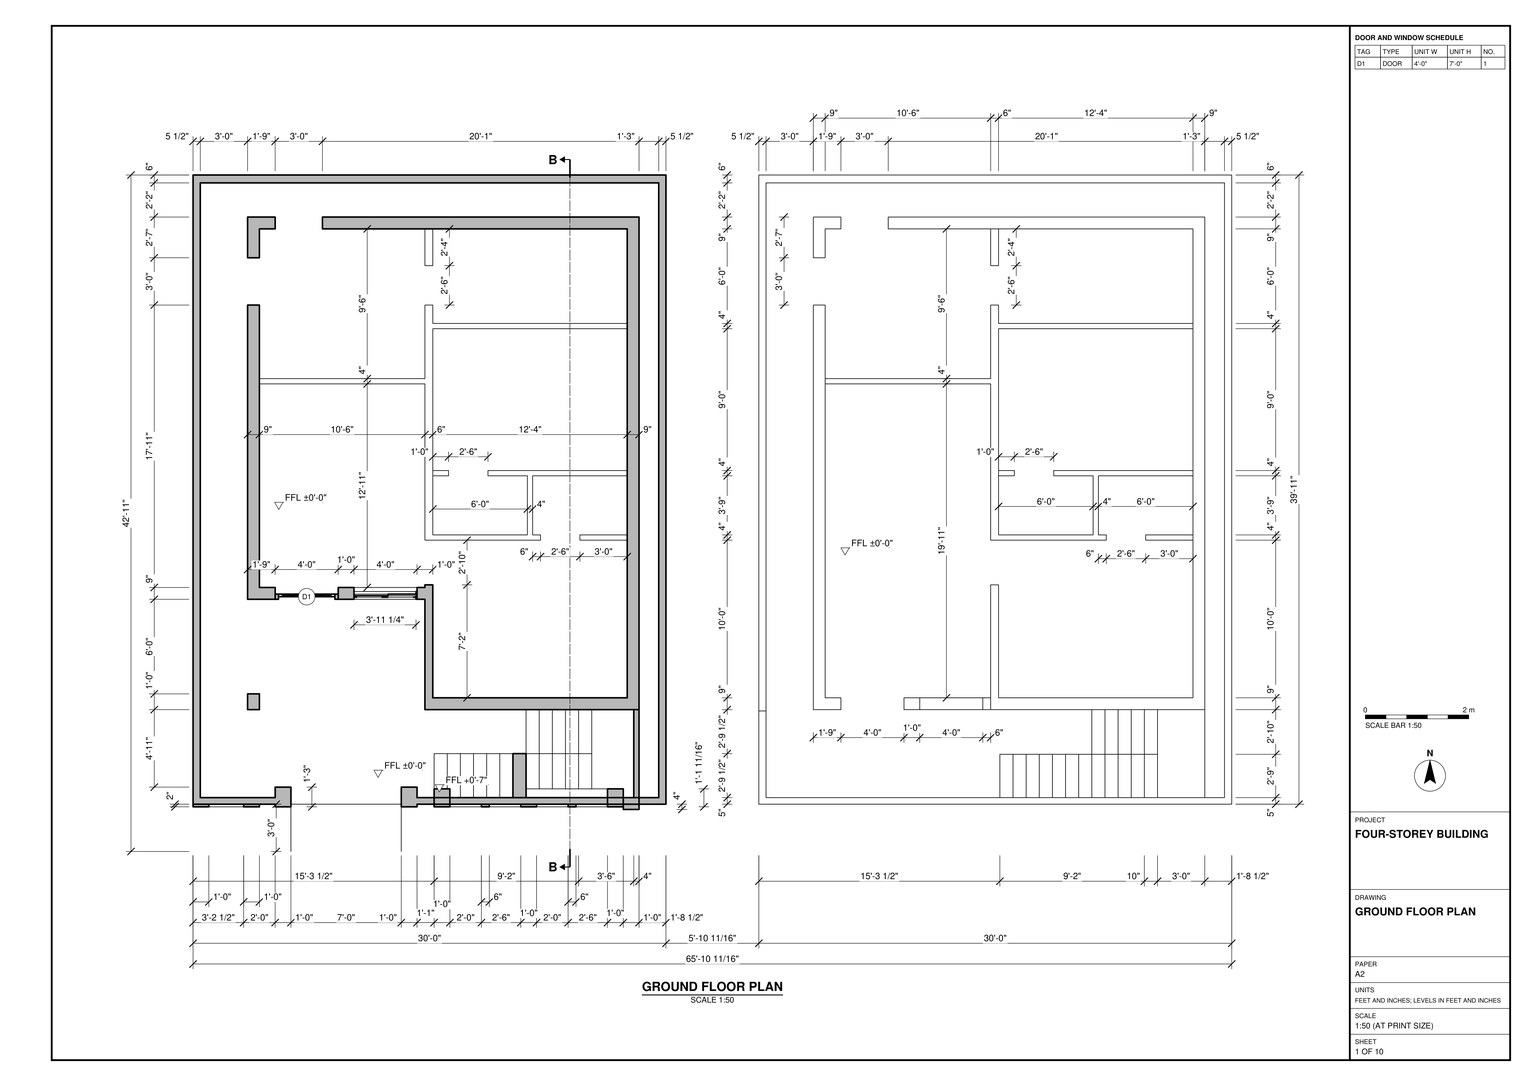
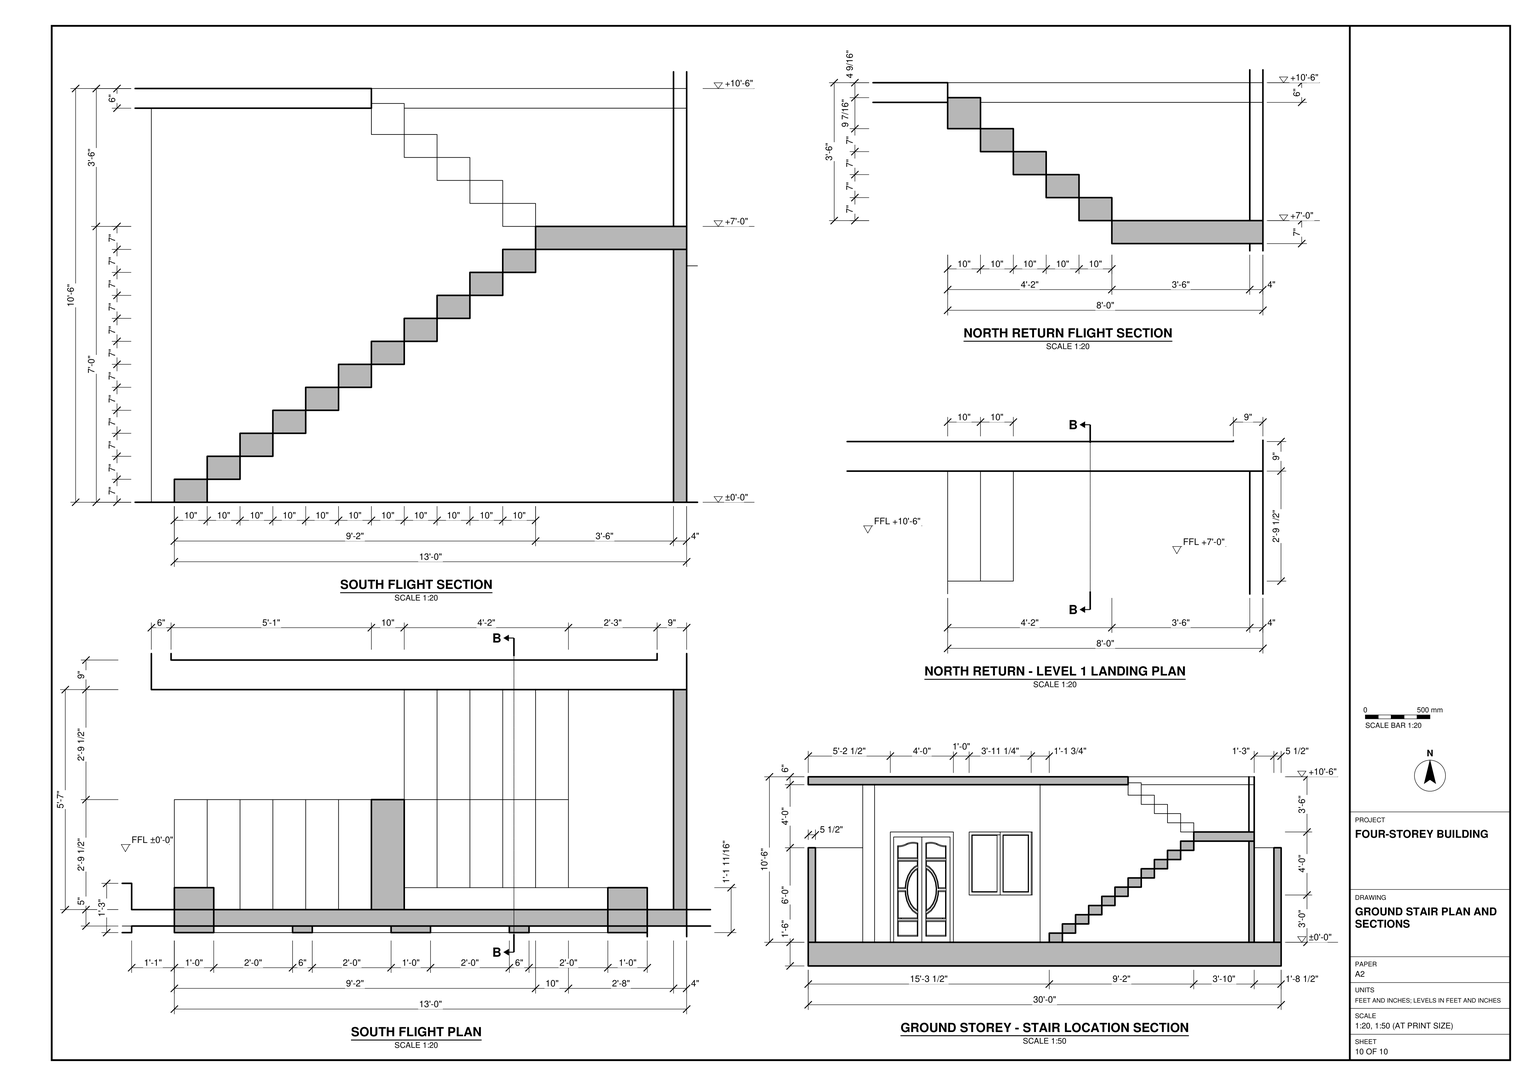
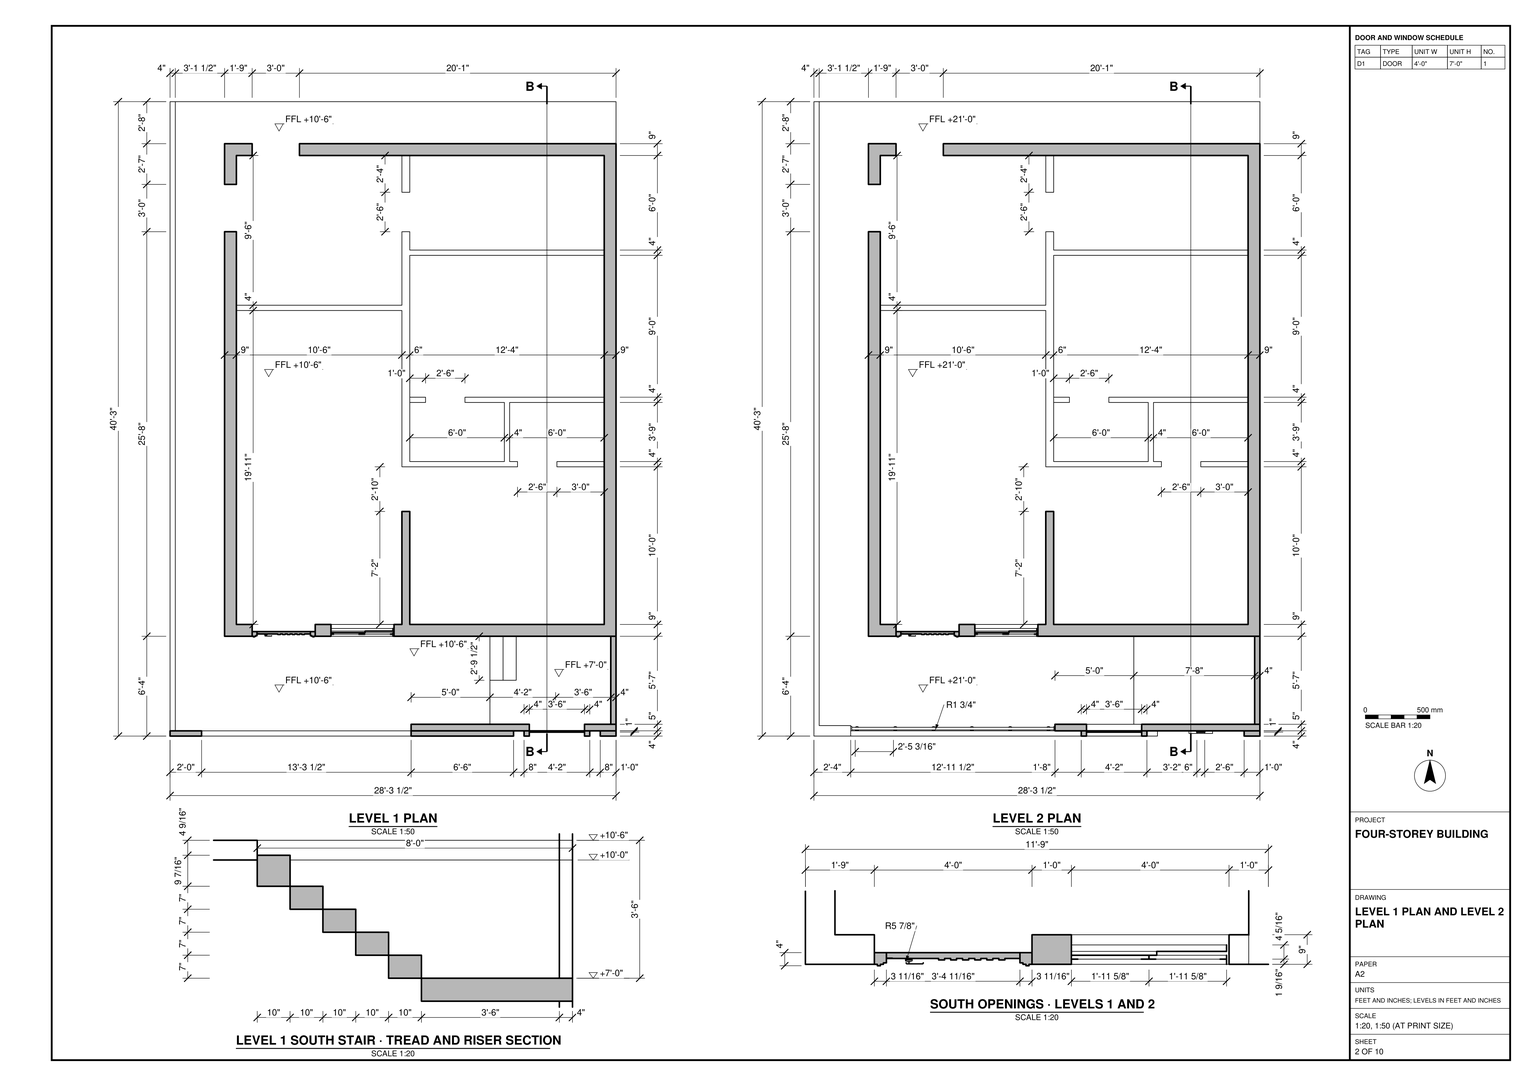
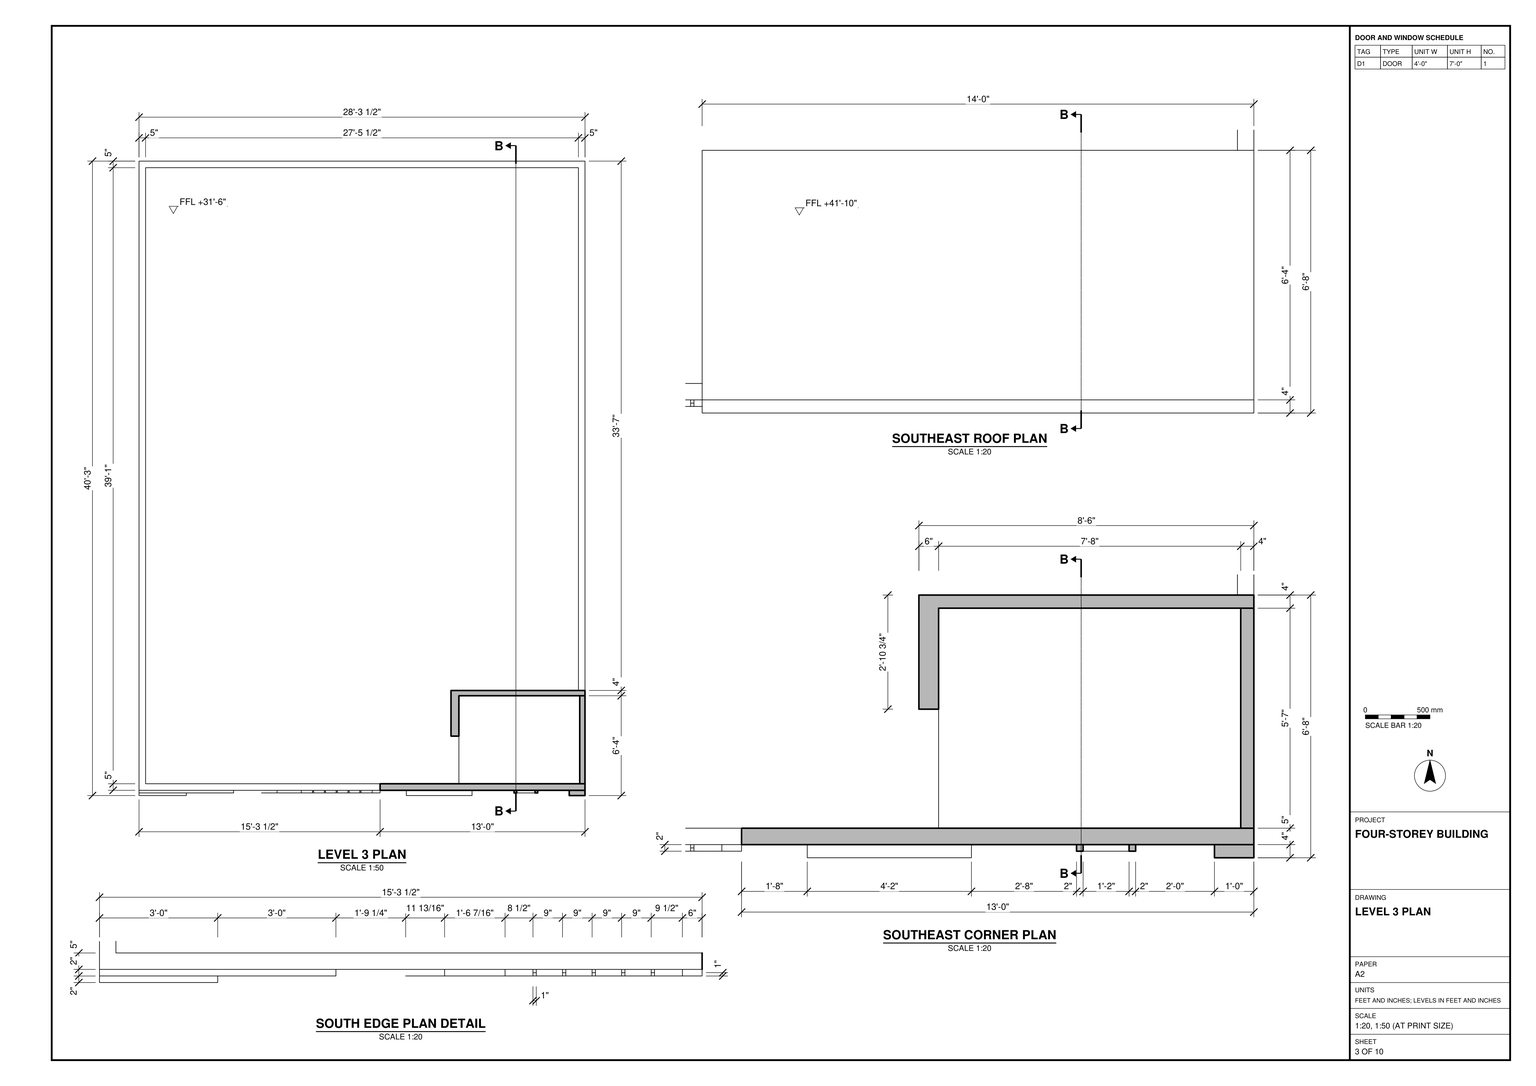
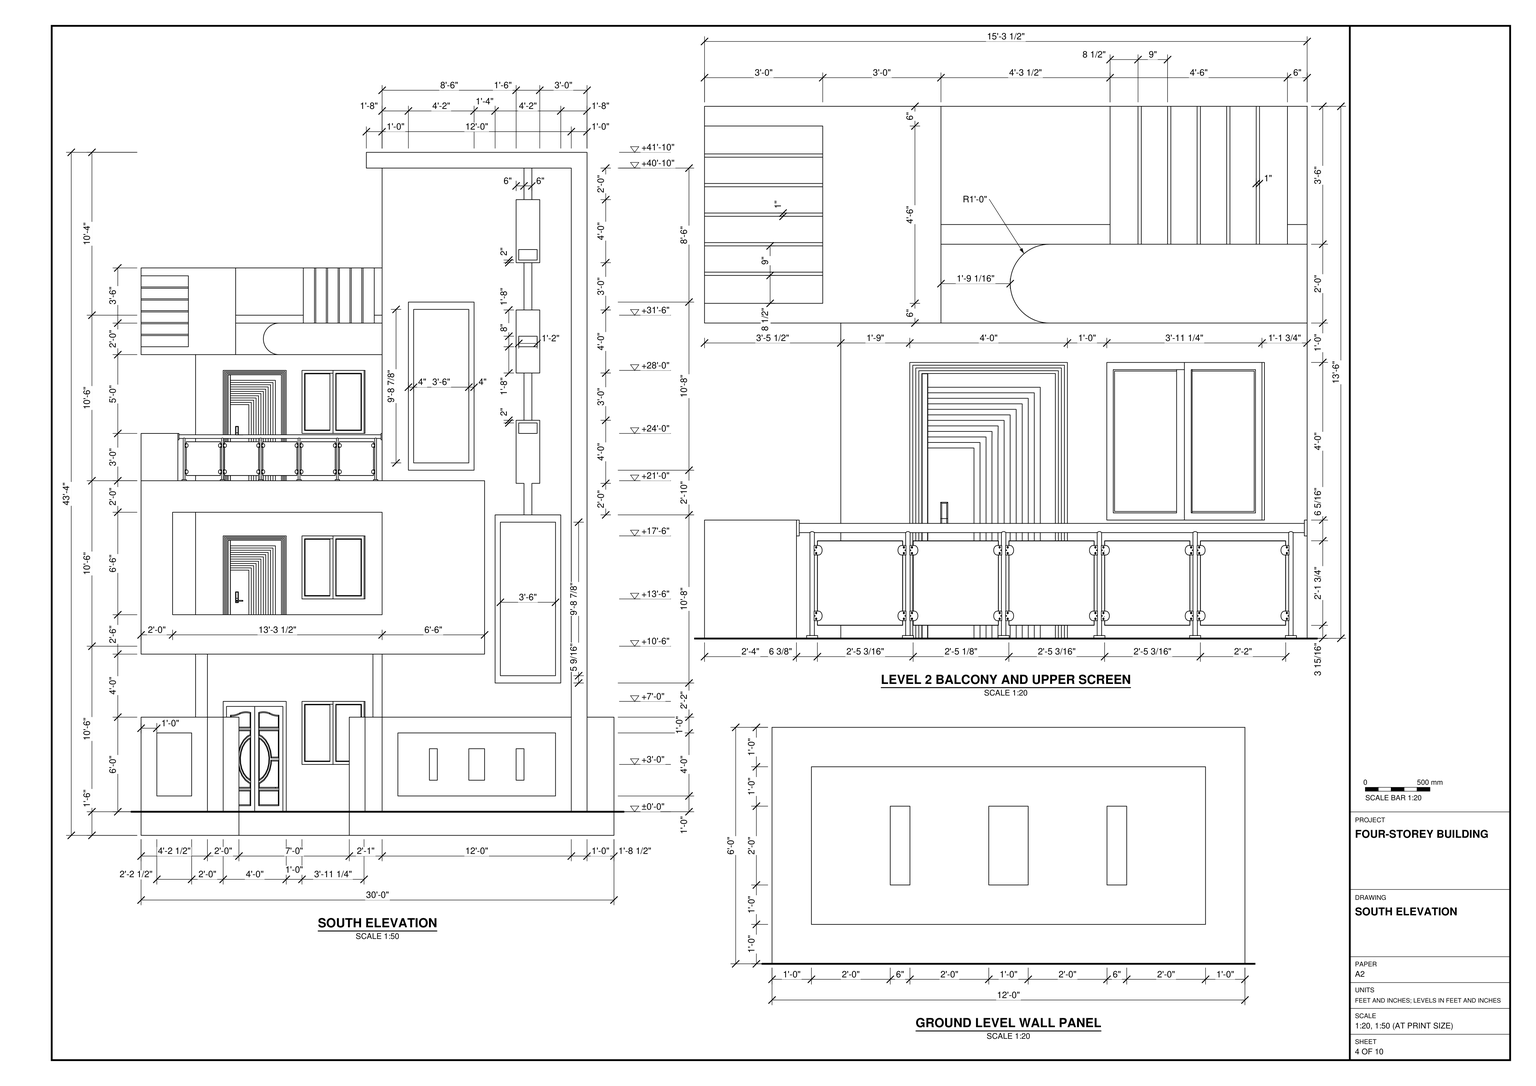
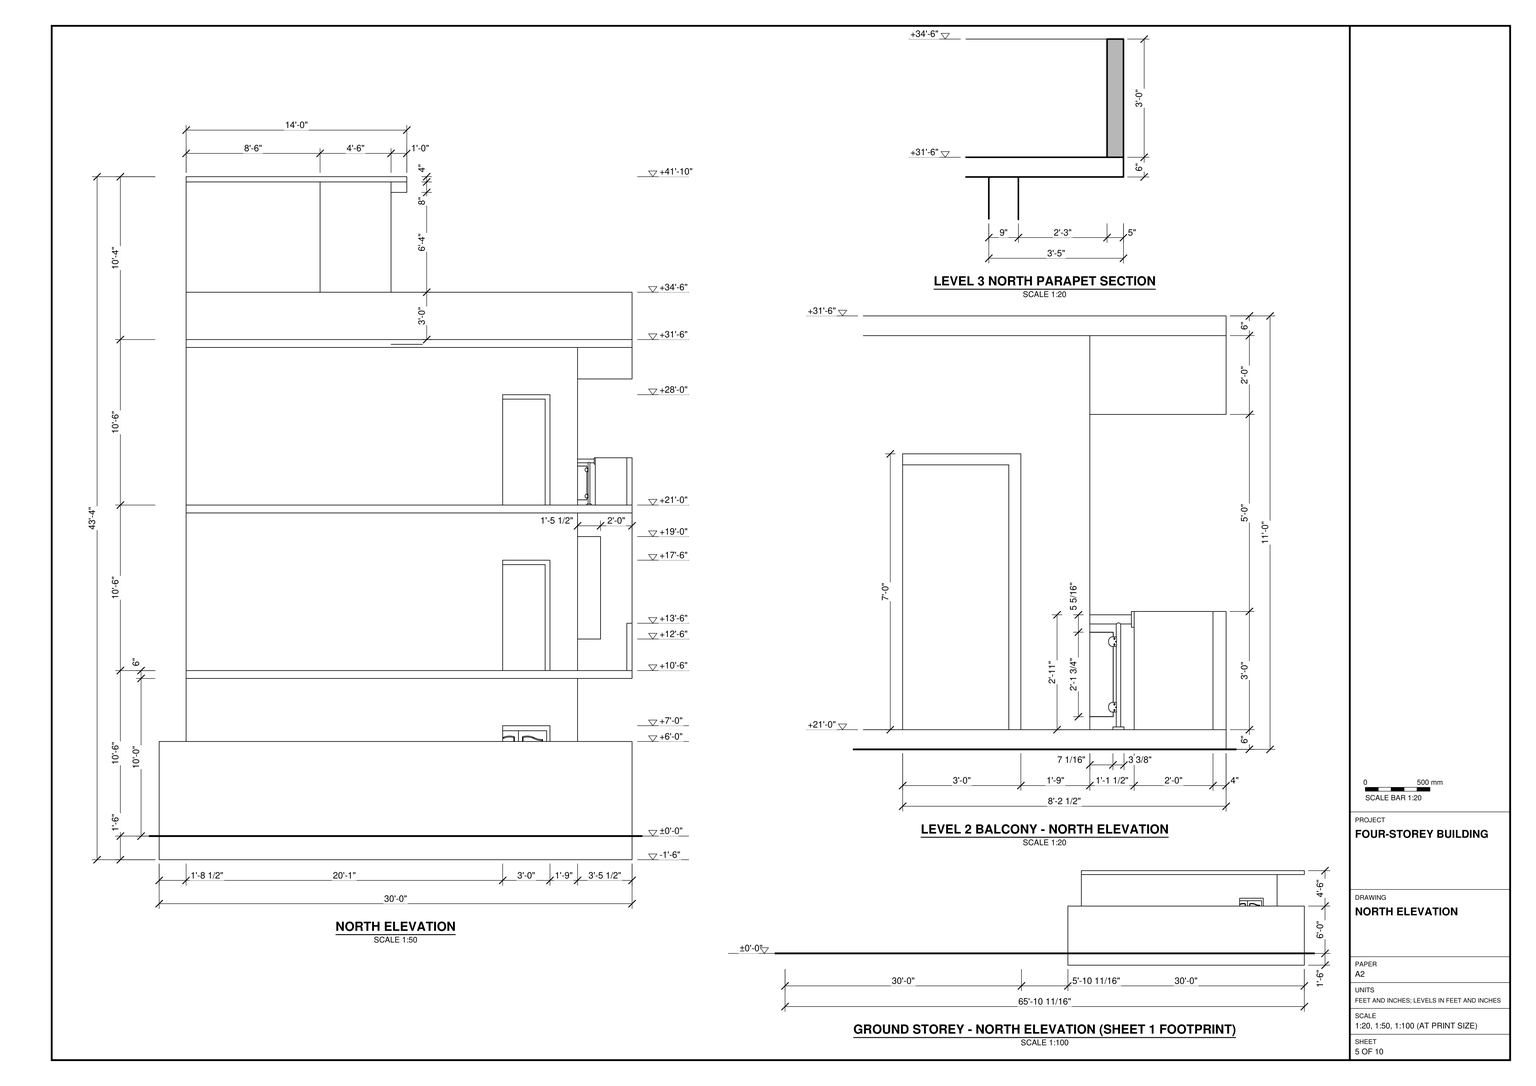
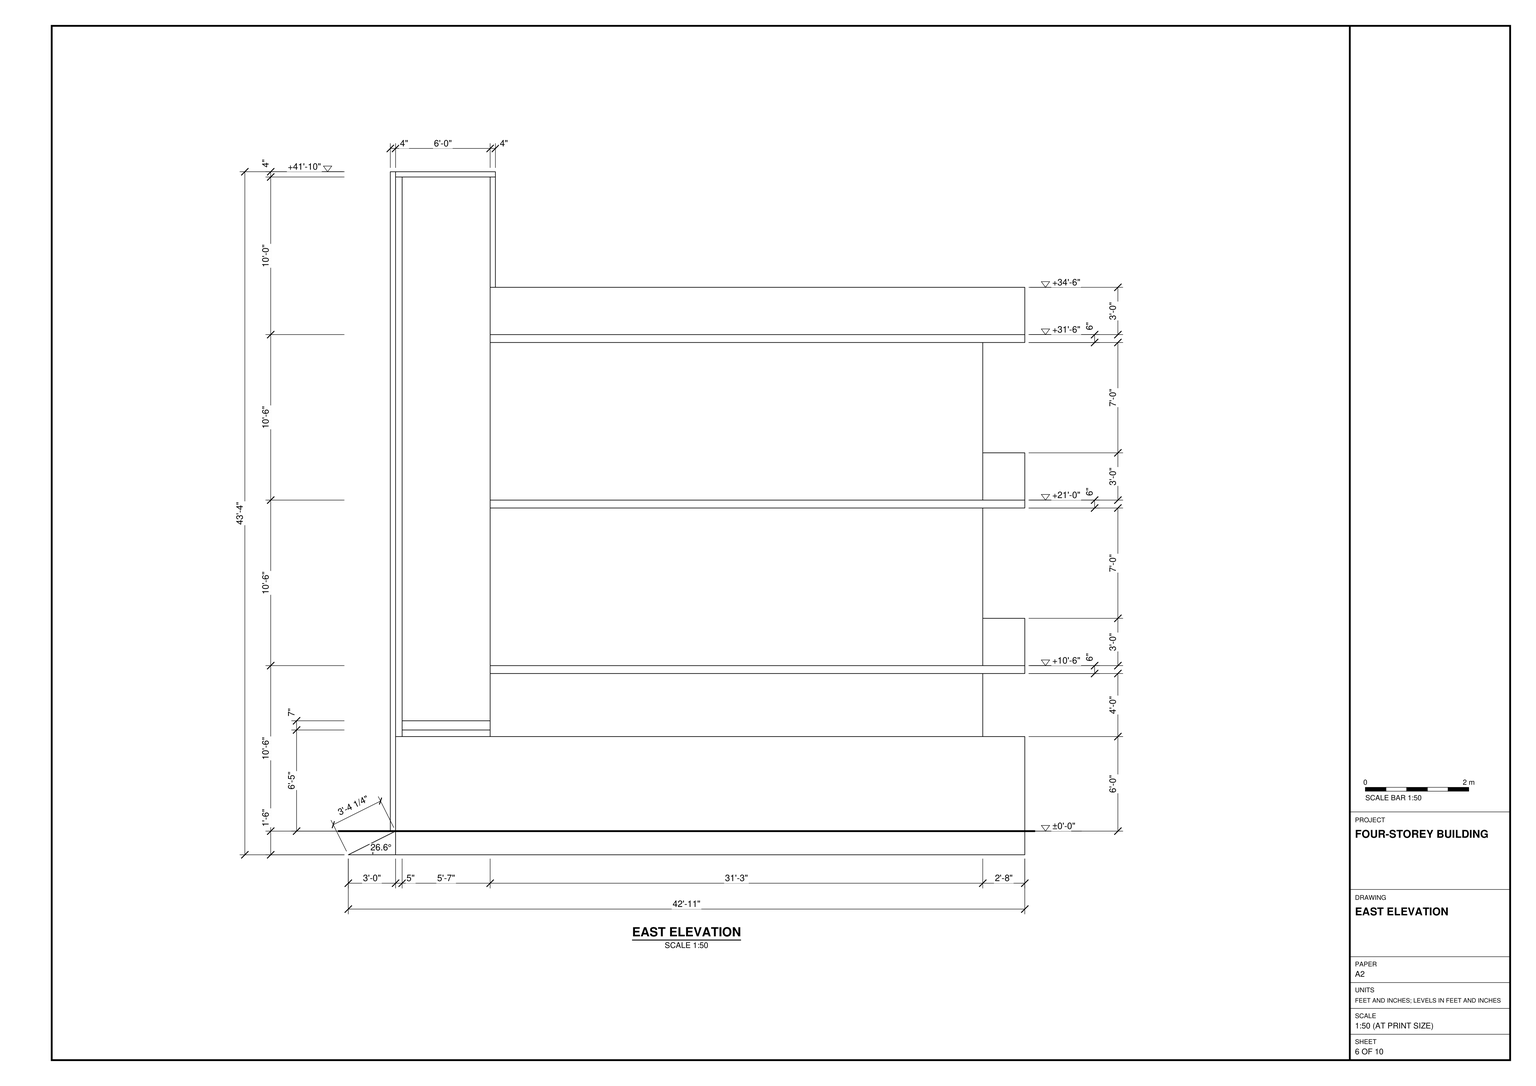
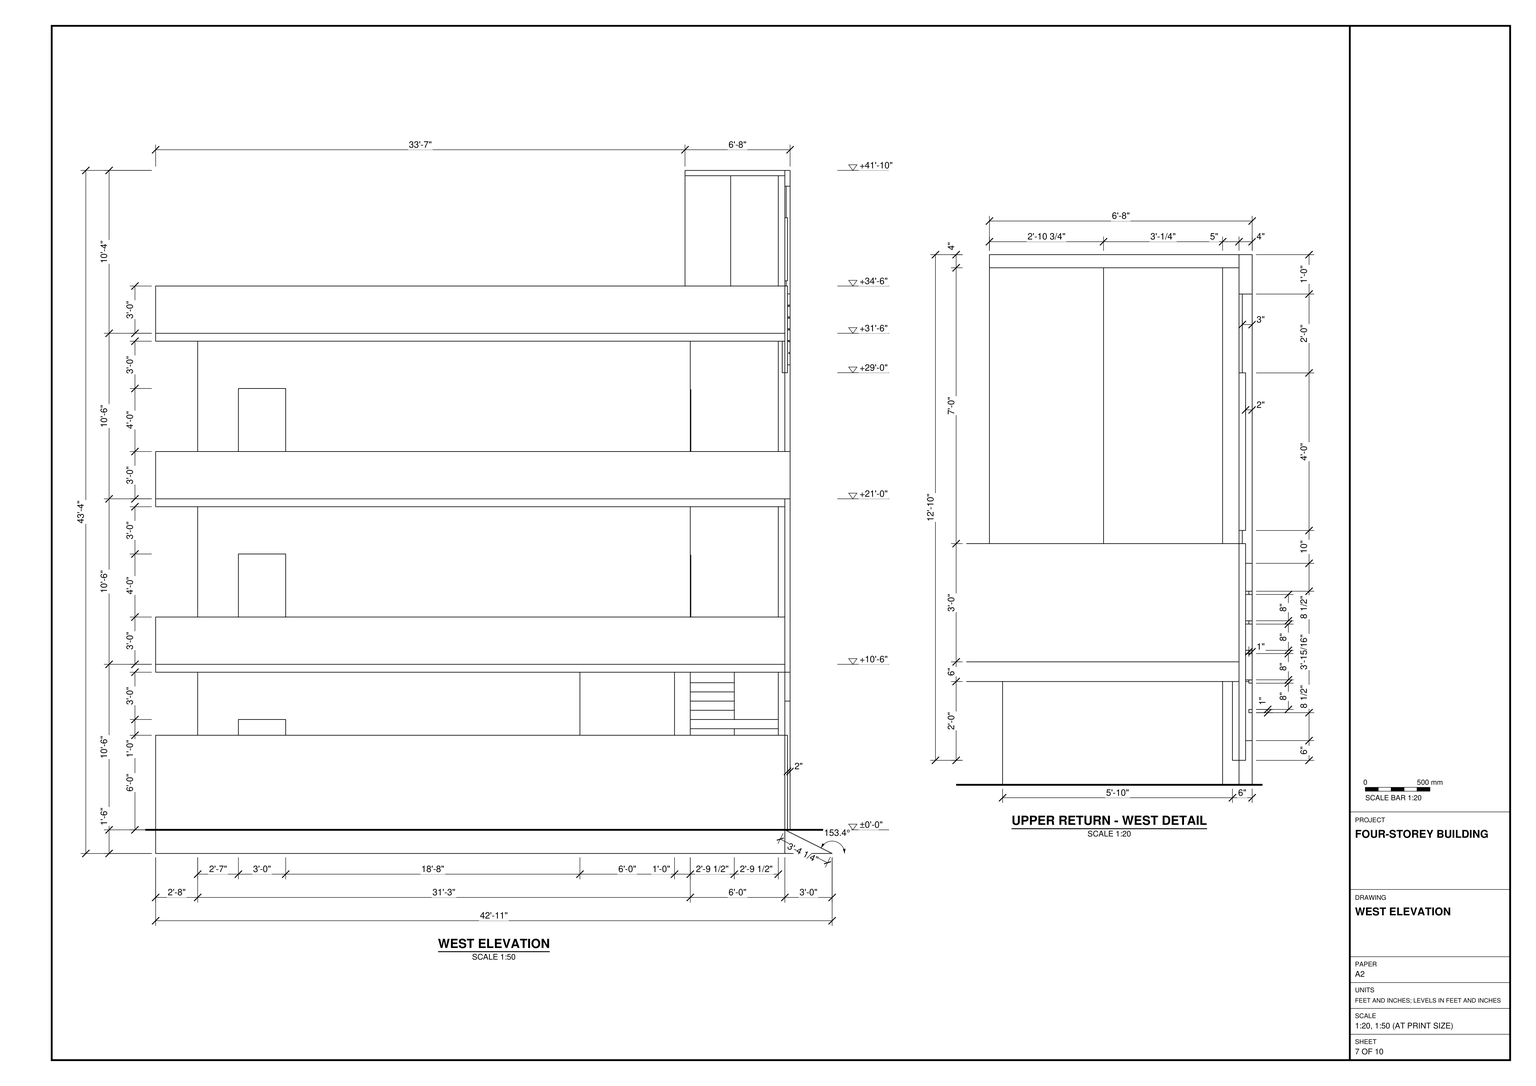
Work in feet and inches. Use task_files/diagram_01.pdf to build the four-storey building in SketchUp. Set out the building on the left and retain the adjacent ground-floor layout to its right, with the 5'-10 11/16" gap shown on the ground-floor plan. The complete model measures 65'-10 11/16" along X, 42'-11" along Y and 43'-4" in height. Set the finished floor levels at ±0'-0", +10'-6", +21'-0" and +31'-6".

Follow each floor plan for the slab outline and wall positions. Preserve the stepped south wall on the ground floor and the exterior floor space in front of the upper-storey openings. Use the wall thicknesses shown, distinguishing the 9" main walls from the 6" and 4" interior walls. Model the doors and window units within their openings. Use the stair sections to build the long south flight, its landing at +7'-0" and the shorter return flight to +10'-6". Coordinate the stair with the opening in the floor slab above. Complete the upper storeys, roof and edge details as drawn, and include built-in joinery and main furniture where shown.

Keep walls, slabs, roof, stairs and individual furniture or joinery pieces in separate groups or components, and use components for repeated parts. Decor and loose items may be any suitable library components. Save one SketchUp model as output_files/four_storey_building_and_its_return_stair.skp.

# SketchUp Ruby script. Lengths in inches.
U = 1.inch
M = Sketchup.active_model
def pt(a) = Geom::Point3d.new(a.map { |v| v * U })
def face(e, loops, mat)
  f = e.add_face(loops[0].map { |a| pt(a) })
  loops[1..].each { |l| e.add_face(l.map { |a| pt(a) }).erase! }
  f.material = f.back_material = mat if mat
  f
end
# faces: each face lists its corners as indices into pts; further lists are holes
def faces(e, pts, list, mat = nil) = list.each { |f| face(e, (f[0].is_a?(Array) ? f : [f]).map { |l| l.map { |i| pts[i] } }, mat) }
# xy, xz, yz: faces in a plane at the given z, y or x. An outline is a flat list of corners, or four numbers for a rectangle; further outlines are holes
def ring(l) = l.size == 4 ? [[l[0], l[1]], [l[2], l[1]], [l[2], l[3]], [l[0], l[3]]] : l.each_slice(2).to_a
def flat(e, list, mat, &to3) = list.each { |f| face(e, (f[0].is_a?(Array) ? f : [f]).map { |l| ring(l).map { |u, v| to3.(u, v) } }, mat) }
def xy(e, z, list, mat = nil) = flat(e, list, mat) { |x, y| [x, y, z] }
def xz(e, y, list, mat = nil) = flat(e, list, mat) { |x, z| [x, y, z] }
def yz(e, x, list, mat = nil) = flat(e, list, mat) { |y, z| [x, y, z] }
def lines(e, pts, list) = list.each { |a, b| e.add_line(pt(pts[a]), pt(pts[b])) }
# prism: a flat outline (further loops are holes) pulled along v
def prism(e, loops, v, mat = nil)
  f = face(e, loops, mat); d = Geom::Vector3d.new(v.map { |x| x * U })
  f.pushpull(f.normal.samedirection?(d) ? d.length : -d.length)
end
def box(e, o, s, mat = nil) = prism(e, [[o, [o[0] + s[0], o[1], o[2]], [o[0] + s[0], o[1] + s[1], o[2]], [o[0], o[1] + s[1], o[2]]]], [0, 0, s[2]], mat)
def at(x, y, z, deg = 0) = Geom::Transformation.translation(pt([x, y, z])) * Geom::Transformation.rotation(ORIGIN, Z_AXIS, deg.degrees)
def axes(o, x, y, z) = Geom::Transformation.new([*x, 0, *y, 0, *z, 0, *pt(o).to_a, 1])
def part(name) = M.definitions.add(name)
# library, detail: a bought-in or finely detailed component or shape, given as its bounding box
def library(name, o, s) = part(name).tap { |d| box(d.entities, o, s) }
def detail(e, o, s) = box(e.add_group.entities, o, s)
def put(e, d, t, mat = nil) = e.add_instance(d, t).tap { |i| i.material = mat if mat }
def group(e, t, mat = nil) = e.add_group.tap { |g| g.transformation = t; g.material = mat if mat }.entities
root = M.entities
M.materials.add("[Translucent Glass Blue]").color = [100, 149, 237]
M.materials["[Translucent Glass Blue]"].alpha = 0.5
c1 = library("Panel balustrade",[0,0,0],[144.88,3.4,25.32])
c2 = library("Single door assembly",[13.9375,0,0],[46.5,4,90])
c3 = library("door+design",[0,0,0],[60.3,3.9375,84])
c4 = part("Janela aluminio")
xy(c4.entities,0,[[0,0,47.24,1.57],[23.62,1.57,47.24,2.76],[0,2.76,25.98,3.9375],[0,3.9375,47.24,5.91]])
xy(c4.entities,43.31,[[0,0,47.24,1.57],[23.62,1.57,47.24,2.76],[0,2.76,0,5.91,47.24,5.91,47.24,3.9375,25.98,3.9375,25.98,2.76],[25.98,2.76,47.24,3.9375]])
xz(c4.entities,1.57,[[0,0,23.62,0,23.62,41.34,21.26,41.34,21.26,1.97,1.97,1.97,1.97,41.34,23.62,41.34,23.62,43.31,0,43.31],[[23.62,0,47.24,43.31],[25.7,1.97,45.28,41.34]]])
xz(c4.entities,2.76,[[[0,0,23.62,43.31],[2.36,2.36,21.26,40.94]],[23.62,0,25.98,43.31]])
xz(c4.entities,2.76,[[2.36,2.36,21.26,40.94]],"[Translucent Glass Blue]")
xz(c4.entities,3.9375,[[25.98,0,25.98,2.36,44.88,2.36,44.88,40.94,25.98,40.94,25.98,43.31,47.24,43.31,47.24,0]])
xz(c4.entities,3.9375,[[25.98,2.36,44.88,40.94]],"[Translucent Glass Blue]")
yz(c4.entities,0,[[0,0,1.57,43.31],[2.76,0,5.91,43.31]])
yz(c4.entities,23.62,[[1.57,0,2.76,43.31]])
yz(c4.entities,25.98,[[2.76,0,3.9375,43.31]])
yz(c4.entities,47.24,[[0,0,1.57,43.31],[1.57,0,2.76,43.31],[3.9375,0,5.91,43.31]])
c5 = part("Group\#8")
box(c5.entities,[0,0,0],[10,33.5,7])
prism(root,[[[183.5,34,372],[105.09,34,372],[104.15,34,371.96],[103.21,34,371.85],[102.29,34,371.67],[101.38,34,371.41],[100.49,34,371.09],[99.64,34,370.69],[98.82,34,370.23],[98.03,34,369.71],[97.29,34,369.125],[96.6,34,368.49],[95.96,34,367.79],[95.38,34,367.05],[94.85,34,366.27],[94.39,34,365.45],[94,34,364.59],[93.67,34,363.71],[93.42,34,362.8],[93.23,34,361.88],[93.125,34,360.94],[93.09,34,360],[93.125,34,359.06],[93.23,34,358.12],[93.42,34,357.2],[93.67,34,356.29],[94,34,355.41],[94.39,34,354.55],[94.85,34,353.73],[95.38,34,352.95],[95.96,34,352.21],[96.6,34,351.51],[97.29,34,350.875],[98.03,34,350.29],[98.82,34,349.77],[99.64,34,349.31],[100.49,34,348.91],[101.38,34,348.59],[102.29,34,348.33],[103.21,34,348.15],[104.15,34,348.04],[105.09,34,348],[183.5,34,348]]],[0,2,0])
box(root,[249.5,34,24],[12,2,24])
box(root,[285.5,34,24],[6,2,24])
box(root,[219.5,34,24],[6,2,24])
p = [[105.09,36,348],[91.75,36,348],[91.75,36,372],[105.09,36,372]]
lines(root,p,[[0,1],[2,3]])
put(root,c1,axes([28,36,252],[1.07329,0,0],[0,1,0],[0,0,1.42174]))
put(root,c2,axes([48.11,107.56,126],[1.03226,0,0],[0,1,0],[0,0,0.93333]))
put(root,c2,axes([48.11,107.56,252],[1.03226,0,0],[0,1,0],[0,0,0.93333]))
put(root,c3,axes([62.5,192,0],[0.79602,0,0],[0,1,0],[0,0,1]))
put(root,c4,axes([122.5,192,36],[1,0,0],[0,1,0],[0,0,1.10836]))
put(root,c4,axes([122.5,108,162],[1,0,0],[0,1,0],[0,0,1.10836]))
put(root,c4,axes([122.5,108,288],[1,0,0],[0,1,0],[0,0,1.10836]))
g1 = group(root,at(430.6875,36,0))
xy(g1,0,[[0,0,360,0,360,479,0,479,0,71,5.5,71,5.5,473,354.5,473,354.5,5,5.5,5,5.5,71,0,71],[[5.5,5,183.5,5,183.5,38,253.5,38,253.5,72,110.5,72,110.5,81,176.5,81,176.5,167,182.5,167,182.5,81,330.5,81,330.5,201,294.5,201,294.5,205,330.5,205,330.5,250,258.5,250,258.5,205,264.5,205,264.5,201,176.5,201,176.5,320,50.5,320,50.5,81,62.5,81,62.5,72,41.5,72,41.5,380,50.5,380,50.5,324,176.5,324,176.5,380,182.5,380,182.5,366,330.5,366,330.5,438,182.5,438,182.5,410,176.5,410,176.5,438,98.5,438,98.5,447,339.5,447,339.5,5,354.5,5,354.5,473,5.5,473],[41.5,416,41.5,447,62.5,447,62.5,438,50.5,438,50.5,416]],[183.5,5,193.5,38],[193.5,5,203.5,38],[203.5,5,213.5,38],
  [213.5,5,223.5,38],[223.5,5,233.5,38],[233.5,5,243.5,38],[243.5,5,253.5,38],[253.5,5,263.5,38],
  [263.5,5,273.5,38],[273.5,5,283.5,38],[283.5,5,293.5,38],[293.5,5,303.5,38],[303.5,5,339.5,72],
  [253.5,38,263.5,72],[263.5,38,273.5,72],[273.5,38,283.5,72],[283.5,38,293.5,72],[293.5,38,303.5,72],
  [41.5,72,62.5,72,62.5,81,50.5,81,50.5,380,41.5,380],[176.5,72,339.5,72,339.5,447,98.5,447,98.5,438,330.5,438,330.5,81,182.5,81,182.5,167,176.5,167],[110.5,72,122.5,81],[122.5,72,170.5,81],[170.5,72,176.5,81],
  [176.5,201,264.5,201,264.5,205,258.5,205,258.5,250,330.5,250,330.5,254,224.5,254,224.5,250,254.5,250,254.5,205,182.5,205,182.5,362,330.5,362,330.5,366,182.5,366,182.5,380,176.5,380,176.5,324,50.5,324,50.5,320,176.5,320],[294.5,201,330.5,205],[182.5,205,254.5,205,254.5,250,224.5,250,224.5,254,330.5,254,330.5,362,182.5,362,182.5,254,194.5,254,194.5,250,182.5,250],[182.5,250,194.5,254],[176.5,410,182.5,438],
  [41.5,416,50.5,416,50.5,438,62.5,438,62.5,447,41.5,447]])
g2 = group(root,at(0,36,0))
xy(g2,0,[[62.5,-2,74.5,-2,74.5,13,62.5,13,62.5,5,5.5,5,5.5,473,354.5,473,354.5,5,339.5,5,339.5,0,360,0,360,479,0,479,0,0,62.5,0],[158.5,-2,170.5,0],[[74.5,0,158.5,0,158.5,13,170.5,13,170.5,5,183.5,5,183.5,38.5,253.5,38.5,253.5,72,176.5,72,176.5,156,110.5,156,110.5,165,176.5,165,176.5,167,182.5,167,182.5,81,330.5,81,330.5,201,294.5,201,294.5,205,330.5,205,330.5,250,258.5,250,258.5,205,264.5,205,264.5,201,176.5,201,176.5,320,50.5,320,50.5,165,62.5,165,62.5,156,41.5,156,41.5,380,50.5,380,50.5,324,176.5,324,176.5,380,182.5,380,182.5,366,330.5,366,330.5,438,182.5,438,182.5,410,176.5,410,176.5,438,98.5,438,98.5,447,339.5,447,339.5,5,354.5,5,354.5,473,5.5,473,5.5,5,62.5,5,62.5,13,74.5,13],[41.5,416,41.5,447,62.5,447,62.5,438,50.5,438,50.5,416],[41.5,72,50.5,84]],[183.5,0,339.5,5],[183.5,5,193.5,38.5],
  [193.5,5,203.5,38.5],[203.5,5,213.5,38.5],[213.5,5,223.5,38.5],[223.5,5,233.5,38.5],[233.5,5,243.5,38.5],
  [243.5,5,253.5,38.5],[253.5,5,263.5,38.5],[263.5,5,273.5,38.5],[273.5,5,283.5,38.5],[283.5,5,293.5,38.5],
  [293.5,5,303.5,38.5],[303.5,5,339.5,72],[253.5,38.5,263.5,72],[263.5,38.5,273.5,72],[273.5,38.5,283.5,72],
  [283.5,38.5,293.5,72],[293.5,38.5,303.5,72],[41.5,72,50.5,84],[176.5,72,339.5,72,339.5,447,98.5,447,98.5,438,330.5,438,330.5,81,182.5,81,182.5,167,176.5,167,176.5,165,170.5,165,170.5,156,176.5,156],[41.5,156,50.5,380],
  [50.5,156,62.5,165],[110.5,156,122.5,165],[122.5,156,170.5,165],[176.5,201,264.5,201,264.5,205,258.5,205,258.5,250,330.5,250,330.5,254,224.5,254,224.5,250,254.5,250,254.5,205,182.5,205,182.5,362,330.5,362,330.5,366,182.5,366,182.5,380,176.5,380,176.5,324,50.5,324,50.5,320,176.5,320],[294.5,201,330.5,205],
  [182.5,205,254.5,205,254.5,250,224.5,250,224.5,254,330.5,254,330.5,362,182.5,362,182.5,254,194.5,254,194.5,250,182.5,250],[182.5,250,194.5,254],[176.5,410,182.5,438],[41.5,416,50.5,416,50.5,438,62.5,438,62.5,447,41.5,447]])
xy(g2,36,[[122.5,156,170.5,165]])
xy(g2,72,[[62.5,-2,74.5,13],[158.5,-2,170.5,13],[0,0,62.5,0,62.5,5,5.5,5,5.5,473,354.5,473,354.5,5,339.5,5,339.5,0,360,0,360,479,0,479],[170.5,0,183.5,5]])
xy(g2,84,[[62.5,156,110.5,165],[122.5,156,170.5,165],[41.5,380,50.5,416],[62.5,438,98.5,447]])
xy(g2,120,[[41.5,72,50.5,84],[176.5,72,339.5,72,339.5,447,62.5,447,62.5,438,330.5,438,330.5,81,182.5,81,182.5,167,176.5,167,176.5,165,170.5,165,170.5,156,176.5,156],[41.5,156,110.5,156,110.5,165,50.5,165,50.5,380,41.5,380],[110.5,156,170.5,165],[41.5,380,50.5,380,50.5,438,62.5,438,62.5,447,41.5,447]])
xz(g2,-2,[[62.5,0,74.5,72],[158.5,0,170.5,72]])
xz(g2,0,[[0,0,62.5,72],[170.5,0,183.5,72],[339.5,0,360,72]])
xz(g2,5,[[5.5,0,62.5,72],[170.5,0,183.5,72],[339.5,0,354.5,72]])
xz(g2,13,[[62.5,0,74.5,72],[158.5,0,170.5,72]])
xz(g2,72,[[41.5,0,50.5,120],[176.5,0,339.5,120]])
xz(g2,81,[[182.5,0,330.5,120]])
xz(g2,84,[[41.5,0,50.5,120]])
xz(g2,156,[[[41.5,0,62.5,0,62.5,84,110.5,84,110.5,0,176.5,0,176.5,120,41.5,120],[122.5,36,170.5,84]]])
xz(g2,165,[[50.5,0,50.5,120,110.5,120,110.5,84,62.5,84,62.5,0],[110.5,0,110.5,120,170.5,120,170.5,84,122.5,84,122.5,0],[122.5,0,170.5,36],[170.5,0,176.5,120]])
xz(g2,167,[[176.5,0,182.5,120]])
xz(g2,380,[[41.5,0,50.5,84]])
xz(g2,416,[[41.5,0,50.5,84]])
xz(g2,438,[[50.5,0,62.5,120],[98.5,0,330.5,0,330.5,120,62.5,120,62.5,84,98.5,84]])
xz(g2,447,[[41.5,0,41.5,120,339.5,120,339.5,0,98.5,0,98.5,84,62.5,84,62.5,0]])
xz(g2,473,[[5.5,0,354.5,72]])
xz(g2,479,[[0,0,360,72]])
yz(g2,0,[[0,0,479,72]])
yz(g2,5.5,[[5,0,473,72]])
yz(g2,41.5,[[72,0,84,120],[156,0,156,120,447,120,447,0,416,0,416,84,380,84,380,0]])
yz(g2,50.5,[[72,0,84,120],[165,0,380,120],[416,0,438,0,438,120,380,120,380,84,416,84]])
yz(g2,62.5,[[-2,0,0,72],[5,0,13,72],[156,0,165,84],[438,0,447,84]])
yz(g2,74.5,[[-2,0,13,72]])
yz(g2,98.5,[[438,0,447,84]])
yz(g2,110.5,[[156,0,165,84]])
yz(g2,122.5,[[156,36,165,84]])
yz(g2,158.5,[[-2,0,13,72]])
yz(g2,170.5,[[-2,0,0,72],[5,0,13,72],[156,36,165,84]])
yz(g2,176.5,[[72,0,156,120],[165,0,167,120]])
yz(g2,182.5,[[81,0,167,120]])
yz(g2,183.5,[[0,0,5,72]])
yz(g2,330.5,[[81,0,438,120]])
yz(g2,339.5,[[0,0,5,72],[72,0,447,120]])
yz(g2,354.5,[[5,0,473,72]])
yz(g2,360,[[0,0,479,72]])
g3 = group(root,at(0,36,126))
xy(g3,0,[[176.5,72,176.5,167,182.5,167,182.5,81,330.5,81,330.5,438,98.5,438,98.5,447,339.5,447,339.5,72],[176.5,201,264.5,201,264.5,205,258.5,205,258.5,250,330.5,250,330.5,254,224.5,254,224.5,250,254.5,250,254.5,205,182.5,205,182.5,362,330.5,362,330.5,366,182.5,366,182.5,380,176.5,380,176.5,324,50.5,324,50.5,320,176.5,320],[294.5,201,330.5,205],[182.5,205,254.5,205,254.5,250,224.5,250,224.5,254,330.5,254,330.5,362,182.5,362,182.5,254,194.5,254,194.5,250,182.5,250],[182.5,250,194.5,254],
  [176.5,410,182.5,438],[41.5,416,41.5,447,62.5,447,62.5,438,50.5,438,50.5,416]])
xy(g3,36,[[122.5,72,170.5,81]])
xy(g3,84,[[62.5,72,110.5,81],[122.5,72,170.5,81],[41.5,380,50.5,416],[62.5,438,98.5,447]])
xy(g3,120,[[41.5,72,339.5,72,339.5,447,62.5,447,62.5,438,330.5,438,330.5,81,182.5,81,182.5,167,176.5,167,176.5,81,50.5,81,50.5,380,41.5,380],[41.5,380,50.5,380,50.5,438,62.5,438,62.5,447,41.5,447]])
xz(g3,72,[[[41.5,0,62.5,0,62.5,84,110.5,84,110.5,0,339.5,0,339.5,120,41.5,120],[122.5,36,170.5,84]]])
xz(g3,81,[[50.5,0,50.5,120,110.5,120,110.5,84,62.5,84,62.5,0],[110.5,0,122.5,120],[122.5,0,170.5,36],[170.5,0,176.5,120],[182.5,0,330.5,120],
  [122.5,84,170.5,120]])
xz(g3,167,[[176.5,0,182.5,120]])
xz(g3,380,[[41.5,0,50.5,84]])
xz(g3,416,[[41.5,0,50.5,84]])
xz(g3,438,[[50.5,0,62.5,120],[98.5,0,330.5,0,330.5,120,62.5,120,62.5,84,98.5,84]])
xz(g3,447,[[41.5,0,41.5,120,339.5,120,339.5,0,98.5,0,98.5,84,62.5,84,62.5,0]])
yz(g3,41.5,[[72,0,72,120,447,120,447,0,416,0,416,84,380,84,380,0]])
yz(g3,50.5,[[81,0,380,120],[416,0,438,0,438,120,380,120,380,84,416,84]])
yz(g3,62.5,[[72,0,81,84],[438,0,447,84]])
yz(g3,98.5,[[438,0,447,84]])
yz(g3,110.5,[[72,0,81,84]])
yz(g3,122.5,[[72,36,81,84]])
yz(g3,170.5,[[72,36,81,84]])
yz(g3,176.5,[[81,0,167,120]])
yz(g3,182.5,[[81,0,167,120]])
yz(g3,330.5,[[81,0,438,120]])
yz(g3,339.5,[[72,0,447,120]])
p = [[0,0,0],[0,479,0]]
lines(g3,p,[[0,1]])
g4 = group(root,at(0,36,252))
xy(g4,0,[[176.5,72,176.5,167,182.5,167,182.5,81,330.5,81,330.5,438,98.5,438,98.5,447,339.5,447,339.5,72],[176.5,201,264.5,201,264.5,205,258.5,205,258.5,250,330.5,250,330.5,254,224.5,254,224.5,250,254.5,250,254.5,205,182.5,205,182.5,362,330.5,362,330.5,366,182.5,366,182.5,380,176.5,380,176.5,324,50.5,324,50.5,320,176.5,320],[294.5,201,330.5,205],[182.5,205,254.5,205,254.5,250,224.5,250,224.5,254,330.5,254,330.5,362,182.5,362,182.5,254,194.5,254,194.5,250,182.5,250],[182.5,250,194.5,254],
  [176.5,410,182.5,438],[41.5,416,41.5,447,62.5,447,62.5,438,50.5,438,50.5,416]])
xy(g4,36,[[122.5,72,170.5,81]])
xy(g4,84,[[62.5,72,110.5,81],[122.5,72,170.5,81],[41.5,380,50.5,416],[62.5,438,98.5,447]])
xy(g4,120,[[41.5,72,339.5,72,339.5,447,62.5,447,62.5,438,330.5,438,330.5,81,182.5,81,182.5,167,176.5,167,176.5,81,50.5,81,50.5,380,41.5,380],[41.5,380,50.5,380,50.5,438,62.5,438,62.5,447,41.5,447]])
xz(g4,72,[[[41.5,0,62.5,0,62.5,84,110.5,84,110.5,0,339.5,0,339.5,120,41.5,120],[122.5,36,170.5,84]]])
xz(g4,81,[[50.5,0,50.5,120,110.5,120,110.5,84,62.5,84,62.5,0],[110.5,0,122.5,120],[122.5,0,170.5,36],[170.5,0,176.5,120],[182.5,0,330.5,120],
  [122.5,84,170.5,120]])
xz(g4,167,[[176.5,0,182.5,120]])
xz(g4,380,[[41.5,0,50.5,84]])
xz(g4,416,[[41.5,0,50.5,84]])
xz(g4,438,[[50.5,0,62.5,120],[98.5,0,330.5,0,330.5,120,62.5,120,62.5,84,98.5,84]])
xz(g4,447,[[41.5,0,41.5,120,339.5,120,339.5,0,98.5,0,98.5,84,62.5,84,62.5,0]])
yz(g4,41.5,[[72,0,72,120,447,120,447,0,416,0,416,84,380,84,380,0]])
yz(g4,50.5,[[81,0,380,120],[416,0,438,0,438,120,380,120,380,84,416,84]])
yz(g4,62.5,[[72,0,81,84],[438,0,447,84]])
yz(g4,98.5,[[438,0,447,84]])
yz(g4,110.5,[[72,0,81,84]])
yz(g4,122.5,[[72,36,81,84]])
yz(g4,170.5,[[72,36,81,84]])
yz(g4,176.5,[[81,0,167,120]])
yz(g4,182.5,[[81,0,167,120]])
yz(g4,330.5,[[81,0,438,120]])
yz(g4,339.5,[[72,0,447,120]])
g5 = group(root,at(293.5,41,77))
box(g5,[0,0,0],[46,67,7])
put(root,c5,at(183.5,41,0))
put(root,c5,at(193.5,41,7))
put(root,c5,at(203.5,41,14))
put(root,c5,at(213.5,41,21))
put(root,c5,at(223.5,41,28))
put(root,c5,at(233.5,41,35))
put(root,c5,at(243.5,41,42))
put(root,c5,at(253.5,41,49))
put(root,c5,at(263.5,41,56))
put(root,c5,at(273.5,41,63))
put(root,c5,at(283.5,41,70))
put(root,c5,at(273.5,74.5,91))
put(root,c5,at(263.5,74.5,98))
put(root,c5,at(253.5,74.5,105))
g6 = group(root,at(243.5,74.5,112))
box(g6,[0,0,0],[10,33.5,9.4375])
g7 = group(root,at(0,36,120))
prism(g7,[[[339.5,479,0],[339.5,72,0],[243.5,72,0],[243.5,5,0],[183.5,5,0],[183.5,0,0],[0,0,0],[0,479,0]]],[0,0,6])
put(root,c5,at(283.5,74.5,84))
g8 = group(root,at(0,36,246))
prism(g8,[[[339.5,479,0],[339.5,72,0],[243.5,72,0],[243.5,5,0],[183.5,5,0],[183.5,0,0],[0,0,0],[0,479,0]]],[0,0,6])
g9 = group(root,at(183.5,36,0))
prism(g9,[[[0,0,0],[156,0,0],[156,0,498],[0,0,498]],[[132,0,103.57],[90,0,103.57],[90,0,222],[132,0,222]],[[24,0,264],[24,0,382.43],[66,0,382.43],[66,0,264]]],[0,5,0])
g10 = group(root,at(335.5,41,0))
box(g10,[0,0,0],[4,67,77])
g11 = group(root,at(335.5,41,84))
box(g11,[0,0,0],[4,67,414])
g12 = group(root,at(0,32,126))
prism(g12,[[[0,0,-6],[261.5,0,-6],[261.5,0,126],[0,0,126]],[[183.5,0,102],[183.5,0,24],[24,0,24],[24,0,102]]],[0,4,0])
g13 = group(root,at(203.5,36,260))
prism(g13,[[[0,0,128],[50,0,128],[50,0,0],[0,0,0]],[[46,0,5.57],[46,0,122.43],[4,0,122.43],[4,0,5.57]]],[0,-4,0])
g14 = group(root,at(269.5,32,98))
prism(g14,[[[0,4,128],[50,4,128],[50,4,0],[0,4,0]],[[4,4,122.43],[4,4,5.57],[46,4,5.57],[46,4,122.43]]],[0,-4,0])
g15 = group(root,at(0,41,252))
prism(g15,[[[28,-9,0],[0,-9,0],[0,474,0],[4,474,0],[4,-1,0],[28,-1,0]]],[0,0,36])
g16 = group(root,at(0,36,126))
box(g16,[0,0,0],[4,479,36])
g17 = group(root,at(273.5,35,103.57),"[Translucent Glass Blue]")
box(g17,[0,0,0],[42,1,118.43])
g18 = group(root,at(207.5,35,264),"[Translucent Glass Blue]")
box(g18,[0,0,0],[42,1,118.43])
g19 = group(root,at(0,36,-18))
xy(g19,0,[[0,0,360,479]])
xz(g19,0,[[0,0,360,18]])
xz(g19,479,[[0,0,360,18]])
yz(g19,0,[[0,0,479,18]])
yz(g19,360,[[0,0,479,18]])
g20 = group(root,at(0,36,378))
prism(g20,[[[183.5,5,0],[183.5,0,0],[0,0,0],[0,479,0],[339.5,479,0],[339.5,72,0],[334.5,72,0],[334.5,474,0],[5,474,0],[5,5,0]]],[0,0,36])
g21 = group(root,at(237.5,77.25,378))
xy(g21,0,[[0,0,0,34.75,97,34.75,97,30.75,6,30.75,6,0]])
xy(g21,36,[[97,30.75,102,34.75]])
xy(g21,120,[[0,0,6,0,6,30.75,102,30.75,102,34.75,0,34.75]])
xz(g21,0,[[0,0,6,120]])
xz(g21,30.75,[[6,0,97,0,97,36,102,36,102,120,6,120]])
xz(g21,34.75,[[0,0,0,120,102,120,102,36,97,36,97,0]])
yz(g21,0,[[0,0,34.75,120]])
yz(g21,6,[[0,0,30.75,120]])
yz(g21,97,[[30.75,0,34.75,36]])
yz(g21,102,[[30.75,36,34.75,120]])
g22 = group(root,at(183.5,41,498))
box(g22,[-12,-5,0],[168,76,4])
g23 = group(root,at(171.5,32,0))
prism(g23,[[[156,4,490],[0,4,490],[0,4,502],[168,4,502],[168,4,0],[156,4,0]]],[0,-4,0])
g24 = group(root,at(0,32,348))
xy(g24,6,[[0,0,36,2]])
xy(g24,14.5,[[0,0,36,1]])
xy(g24,15.5,[[0,0,36,1]])
xy(g24,23.5,[[0,0,36,1]])
xy(g24,24.5,[[0,0,36,1]])
xy(g24,32.5,[[0,0,36,1]])
xy(g24,33.5,[[0,0,36,1]])
xy(g24,41.5,[[0,0,36,1]])
xy(g24,42.5,[[0,0,36,1]])
xy(g24,50.5,[[0,0,36,1]])
xy(g24,51.5,[[0,0,36,1]])
xy(g24,60,[[0,0,36,2]])
xz(g24,0,[[0,6,36,14.5],[0,15.5,36,23.5],[0,24.5,36,32.5],[0,33.5,36,41.5],[0,42.5,36,50.5],
  [0,51.5,36,60]])
xz(g24,1,[[0,14.5,36,15.5],[0,23.5,36,24.5],[0,32.5,36,33.5],[0,41.5,36,42.5],[0,50.5,36,51.5]])
xz(g24,2,[[0,6,2,24]])
yz(g24,0,[[0,6,0,14.5,1,14.5,1,15.5,0,15.5,0,23.5,1,23.5,1,24,2,24,2,6],[1,24,2,24.5],[0,24.5,2,32.5],[1,32.5,2,33.5],[0,33.5,2,41.5],
  [1,41.5,2,42.5],[0,42.5,2,50.5],[1,50.5,2,51.5],[0,51.5,2,60]])
yz(g24,36,[[0,6,2,14.5],[1,14.5,2,15.5],[0,15.5,2,23.5],[1,23.5,2,24.5],[0,24.5,2,32.5],
  [1,32.5,2,33.5],[0,33.5,2,41.5],[1,41.5,2,42.5],[0,42.5,2,50.5],[1,50.5,2,51.5],
  [0,51.5,2,60]])
g25 = group(root,at(0,34,354))
box(g25,[0,0,-6],[72,2,66])
g26 = group(root,at(0,36,372))
prism(g26,[[[339.5,479,0],[339.5,72,0],[243.5,72,0],[243.5,5,0],[183.5,5,0],[183.5,0,0],[0,0,0],[0,479,0]]],[0,0,6])
g27 = group(root,at(0,36,348))
box(g27,[0,0,0],[183.5,2,24])
g28 = group(root,at(183.5,34,372))
xy(g28,0,[[-60,0,-51.5,2],[-50.5,0,-42.5,2],[-41.5,0,-33.5,2],[-32.5,0,-24.5,2],[-23.5,0,-23.5,1,-24,1,-24,2,-6,2,-6,0,-14.5,0,-14.5,1,-15.5,1,-15.5,0],
  [-51.5,1,-50.5,2],[-42.5,1,-41.5,2],[-33.5,1,-32.5,2],[-24.5,1,-24,2]])
xy(g28,42,[[-60,0,-51.5,2],[-50.5,0,-42.5,2],[-41.5,0,-33.5,2],[-32.5,0,-24.5,2],[-23.5,0,-15.5,2],
  [-14.5,0,-6,2],[-51.5,1,-50.5,2],[-42.5,1,-41.5,2],[-33.5,1,-32.5,2],[-24.5,1,-23.5,2],
  [-15.5,1,-14.5,2]])
xz(g28,0,[[-60,0,-51.5,42],[-50.5,0,-42.5,42],[-41.5,0,-33.5,42],[-32.5,0,-24.5,42],[-23.5,0,-15.5,42],
  [-14.5,0,-6,42]])
xz(g28,1,[[-51.5,0,-50.5,42],[-42.5,0,-41.5,42],[-33.5,0,-32.5,42],[-24.5,0,-23.5,42],[-15.5,0,-14.5,42]])
xz(g28,2,[[-24,0,-6,2.33]])
yz(g28,-60,[[0,0,2,42]])
yz(g28,-51.5,[[0,0,1,42]])
yz(g28,-50.5,[[0,0,1,42]])
yz(g28,-42.5,[[0,0,1,42]])
yz(g28,-41.5,[[0,0,1,42]])
yz(g28,-33.5,[[0,0,1,42]])
yz(g28,-32.5,[[0,0,1,42]])
yz(g28,-24.5,[[0,0,1,42]])
yz(g28,-23.5,[[0,0,1,42]])
yz(g28,-15.5,[[0,0,1,42]])
yz(g28,-14.5,[[0,0,1,42]])
yz(g28,-6,[[0,0,2,42]])
p = [[-24,481,2.33],[0,481,2.33]]
lines(g28,p,[[0,1]])
g29 = group(root,at(285.5,34,226))
xy(g29,0,[[6,0,12,2]])
xy(g29,24,[[0,0,6,2],[12,0,18,2]])
xy(g29,62,[[2,0,6,2],[6,0,12,2],[12,0,16,2]])
xy(g29,70,[[2,0,6,2],[6,0,12,2],[12,0,16,2]])
xy(g29,72,[[0,0,6,2],[6,0,12,1],[12,0,18,2]])
xy(g29,108,[[0,0,6,2],[6,0,12,1],[12,0,18,2]])
xy(g29,128,[[2,0,16,2]])
xy(g29,136,[[2,0,16,2]])
xy(g29,156,[[0,0,6,2],[6,0,12,1],[12,0,18,2]])
xy(g29,192,[[0,0,6,2],[6,0,12,1],[12,0,18,2]])
xy(g29,194,[[2,0,16,2]])
xy(g29,202,[[2,0,16,2]])
xy(g29,240,[[0,0,6,2],[6,0,12,1],[12,0,18,2]])
xy(g29,264,[[6,1,12,2]])
xz(g29,0,[[[6,0,12,0,12,24,18,24,18,72,0,72,0,24,6,24],[2,62,16,70]],[[0,108,18,156],[2,128,16,136]],[[0,192,18,240],[2,194,16,202]]])
xz(g29,1,[[6,72,12,108],[6,156,12,192],[6,240,12,264]])
xz(g29,2,[[0,24,6,60],[12,24,18,60],[2,62,16,70],[12,108,18,126],[0,138,6,156],
  [12,138,18,156],[0,204,6,240],[12,204,18,240]])
yz(g29,0,[[0,24,2,72],[0,108,2,156],[0,192,2,240]])
yz(g29,2,[[0,62,2,70],[0,128,2,136],[0,194,2,202]])
yz(g29,6,[[0,0,2,24],[1,72,2,108],[1,156,2,192],[1,240,2,264]])
yz(g29,12,[[0,0,2,24],[1,72,2,108],[1,156,2,192],[1,240,2,264]])
yz(g29,16,[[0,62,2,70],[0,128,2,136],[0,194,2,202]])
yz(g29,18,[[0,24,2,72],[0,108,2,156],[0,192,2,240]])
g30 = group(root,at(183.5,34,0))
xy(g30,0,[[0,0,144,13.6875]])
xy(g30,12,[[12,0,132,2],[12,2,132,13.6875]])
xy(g30,60,[[12,0,132,2],[12,2,132,13.6875]])
xy(g30,72,[[0,0,144,13.6875]])
xz(g30,0,[[[0,0,144,72],[12,12,132,60]]])
xz(g30,2,[[12,12,132,60]])
xz(g30,13.6875,[[[0,0,144,72],[12,12,132,60]]])
yz(g30,0,[[0,0,13.6875,72]])
yz(g30,12,[[0,12,2,60],[2,12,13.6875,60]])
yz(g30,132,[[0,12,2,60],[2,12,13.6875,60]])
yz(g30,144,[[0,0,13.6875,72]])
g31 = group(root,at(0,34,0))
xy(g31,0,[[0,0,50.5,2]])
xy(g31,12,[[12,0,38.5,2]])
xy(g31,60,[[12,0,38.5,2]])
xy(g31,72,[[0,0,50.5,2]])
xz(g31,0,[[[0,0,50.5,72],[12,12,38.5,60]]])
xz(g31,2,[[[0,0,50.5,72],[12,12,38.5,60]],[12,12,38.5,60]])
yz(g31,0,[[0,0,2,72]])
yz(g31,12,[[0,12,2,60]])
yz(g31,38.5,[[0,12,2,60]])
yz(g31,50.5,[[0,0,2,72]])
p = [[62.5,2,0],[62.5,2,72],[50.5,2,72],[50.5,2,0]]
lines(g31,p,[[0,1],[1,2],[3,0]])
g32 = group(root,at(74.5,0,-18))
prism(g32,[[[0,36,0],[0,0,0],[0,36,18]]],[84,0,0])
